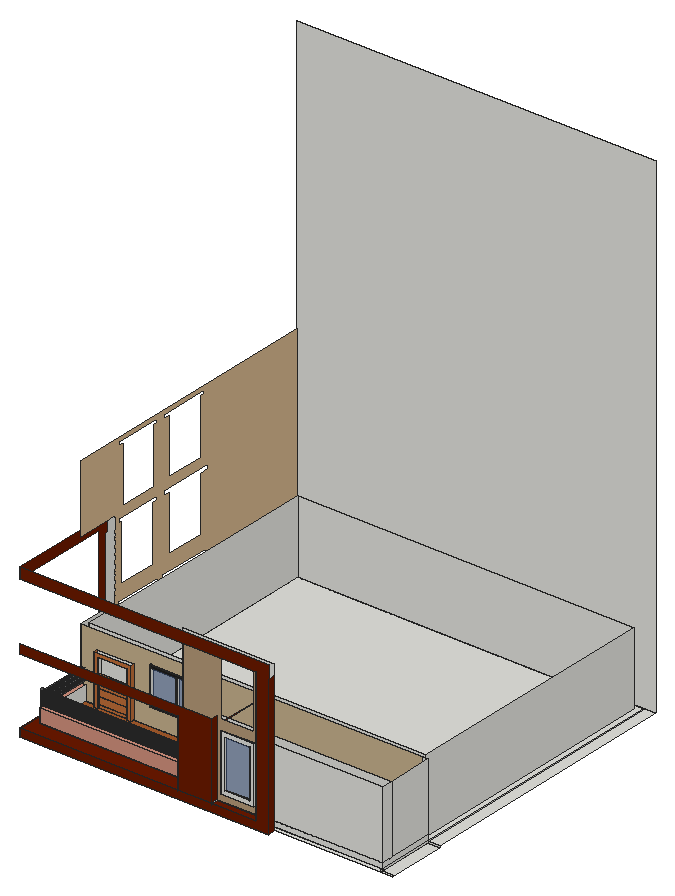
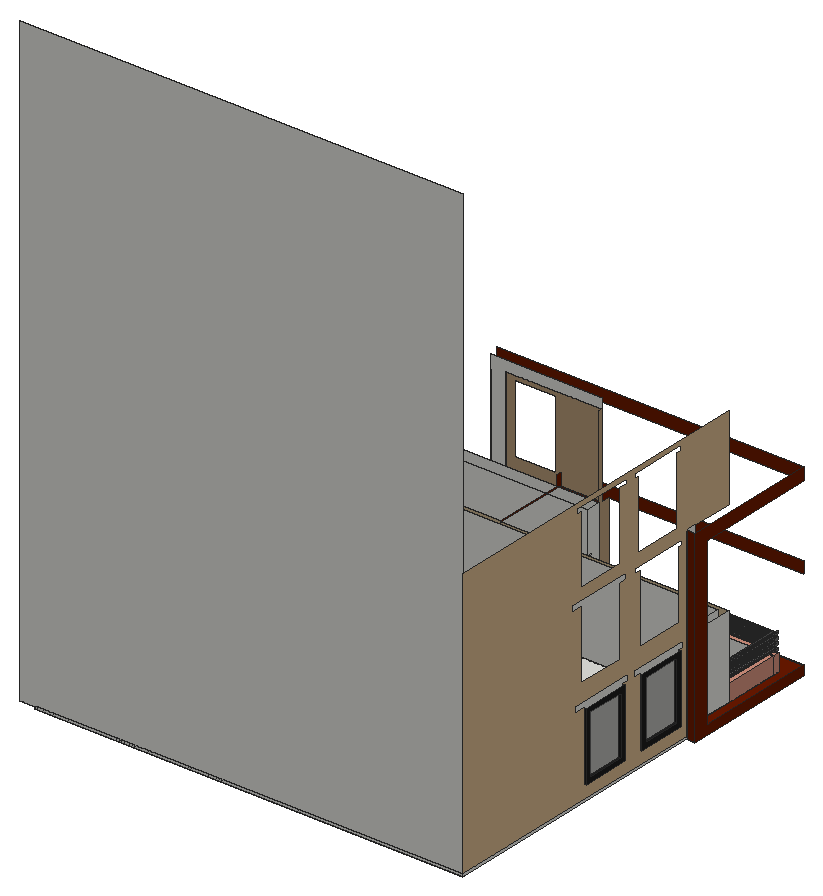
# SketchUp Ruby script. Lengths in inches.
U = 1.inch
M = Sketchup.active_model
def pt(a) = Geom::Point3d.new(a.map { |v| v * U })
def face(e, loops, mat)
  f = e.add_face(loops[0].map { |a| pt(a) })
  loops[1..].each { |l| e.add_face(l.map { |a| pt(a) }).erase! }
  f.material = f.back_material = mat if mat
  f
end
# faces: each face lists its corners as indices into pts; further lists are holes
def faces(e, pts, list, mat = nil) = list.each { |f| face(e, (f[0].is_a?(Array) ? f : [f]).map { |l| l.map { |i| pts[i] } }, mat) }
# xy, xz, yz: faces in a plane at the given z, y or x. An outline is a flat list of corners, or four numbers for a rectangle; further outlines are holes
def ring(l) = l.size == 4 ? [[l[0], l[1]], [l[2], l[1]], [l[2], l[3]], [l[0], l[3]]] : l.each_slice(2).to_a
def flat(e, list, mat, &to3) = list.each { |f| face(e, (f[0].is_a?(Array) ? f : [f]).map { |l| ring(l).map { |u, v| to3.(u, v) } }, mat) }
def xy(e, z, list, mat = nil) = flat(e, list, mat) { |x, y| [x, y, z] }
def xz(e, y, list, mat = nil) = flat(e, list, mat) { |x, z| [x, y, z] }
def yz(e, x, list, mat = nil) = flat(e, list, mat) { |y, z| [x, y, z] }
def lines(e, pts, list) = list.each { |a, b| e.add_line(pt(pts[a]), pt(pts[b])) }
# prism: a flat outline (further loops are holes) pulled along v
def prism(e, loops, v, mat = nil)
  f = face(e, loops, mat); d = Geom::Vector3d.new(v.map { |x| x * U })
  f.pushpull(f.normal.samedirection?(d) ? d.length : -d.length)
end
def box(e, o, s, mat = nil) = prism(e, [[o, [o[0] + s[0], o[1], o[2]], [o[0] + s[0], o[1] + s[1], o[2]], [o[0], o[1] + s[1], o[2]]]], [0, 0, s[2]], mat)
def at(x, y, z, deg = 0) = Geom::Transformation.translation(pt([x, y, z])) * Geom::Transformation.rotation(ORIGIN, Z_AXIS, deg.degrees)
def axes(o, x, y, z) = Geom::Transformation.new([*x, 0, *y, 0, *z, 0, *pt(o).to_a, 1])
def part(name) = M.definitions.add(name)
# library, detail: a bought-in or finely detailed component or shape, given as its bounding box
def library(name, o, s) = part(name).tap { |d| box(d.entities, o, s) }
def detail(e, o, s) = box(e.add_group.entities, o, s)
def put(e, d, t, mat = nil) = e.add_instance(d, t).tap { |i| i.material = mat if mat }
def group(e, t, mat = nil) = e.add_group.tap { |g| g.transformation = t; g.material = mat if mat }.entities
root = M.entities
M.materials.add("[0032_Moccasin]").color = [198, 177, 141]
M.materials.add("[0035_Tan]").color = [181, 154, 120]
M.materials.add("[0035_Tan]1").color = [210, 180, 140]
M.materials.add("[0134_DimGray]").color = [105, 105, 105]
M.materials.add("[Color B02]").color = [209, 145, 125]
M.materials.add("[Color B07]").color = [107, 26, 0]
M.materials.add("[Color M08]").color = [30, 30, 30]
M.materials.add("[Translucent Glass Blue]").color = [61, 91, 145]
M.materials["[Translucent Glass Blue]"].alpha = 0.5
M.materials.add("[Translucent Glass Gray]").color = [128, 128, 128]
M.materials["[Translucent Glass Gray]"].alpha = 0.5
M.materials.add("[Wood Square Tile 01]").color = [164, 91, 44]
M.materials.add("[Wood Veneer 01]").color = [191, 111, 58]
xy(root,123,[[[23.624,9.857,23.624,189.6875,34.874,189.6875,34.874,561.976,604.124,561.976,604.124,23.9375,299.436,23.9375,299.436,20.9375,430.624,20.9375,430.624,9.857],[542.499,503.926,551.499,532.164],[542.499,420.614,551.499,448.851],[542.499,52.1875,551.499,80.425]],[604.124,23.9375,622.998,26.9375],[604.124,26.9375,622.998,119.9375],[542.499,52.1875,551.499,80.425],[542.499,503.926,551.499,532.164]])
xy(root,126,[[34.874,26.9375,410.072,35.9375],[410.072,26.9375,410.072,35.9375,595.124,35.9375,595.124,119.9375,604.124,119.9375,604.124,26.9375],[34.874,35.9375,34.874,119.9375,61.398,119.9375,61.398,113.9375,67.398,113.9375,67.398,116.9375,115.398,116.9375,115.398,113.9375,121.398,113.9375,121.398,119.9375,595.124,119.9375,595.124,35.9375],[61.398,113.9375,67.398,119.9375],[115.398,113.9375,121.398,119.9375],
  [67.398,116.9375,115.398,119.9375],[34.874,119.9375,38.249,189.6875],[[38.249,119.9375,604.124,119.9375,604.124,561.976,34.874,561.976,34.874,189.6875,38.249,189.6875],[43.874,125.9375,595.124,552.976]],[604.124,119.9375,622.998,561.976],[43.874,125.9375,595.124,552.976]])
xy(root,134.528,[[282.124,16.419,337.624,20.9375],[282.124,20.9375,410.072,26.9375],[410.072,26.9375,604.124,26.9375,604.124,44.9375,595.124,44.9375,595.124,35.9375,410.072,35.9375],[410.072,35.9375,595.124,44.9375]])
xy(root,134.528,[[43.874,44.9375,604.124,44.9375,604.124,119.9375,121.398,119.9375,121.398,113.9375,115.398,113.9375,115.398,116.9375,67.398,116.9375,67.398,113.9375,61.398,113.9375,61.398,119.9375,43.874,119.9375]],"[Wood Square Tile 01]")
xy(root,136.146,[[282.124,9.857,337.624,20.9375],[282.124,26.9375,410.072,35.9375],[34.874,35.9375,38.249,44.9375],[38.249,35.9375,282.124,44.9375],[282.124,35.9375,410.072,44.9375]])
xy(root,136.146,[[23.624,9.857,282.124,9.857,282.124,35.9375,34.874,35.9375,34.874,170.669,23.624,170.669],[337.624,9.857,410.072,20.9375]],"[Color B07]")
xy(root,144.554,[[31.874,203.038,34.874,267.163],[31.874,295.913,34.874,360.038]],"[Color M08]")
xy(root,149.334,[[346.097,17.9375,399.784,20.9375]])
xy(root,150.554,[[31.874,209.038,34.874,261.163],[31.874,301.913,34.874,354.038]],"[Color M08]")
xy(root,155.334,[[352.097,17.9375,393.784,20.9375]])
xy(root,158.528,[[410.072,35.9375,595.124,44.9375]])
xy(root,158.528,[[34.874,35.9375,410.072,44.9375],[34.874,44.9375,43.874,119.9375]],"[Color B02]")
xy(root,165.189,[[149.96,116.9375,235.647,119.9375]])
xy(root,168.189,[[152.96,116.9375,192.804,119.9375],[195.804,116.9375,232.647,119.9375]])
xz(root,9.857,[[23.624,123,430.624,123,430.624,372,23.624,372,23.624,355.125,410.072,355.125,410.072,136.146,23.624,136.146],[282.124,136.146,337.624,136.146,337.624,260.108,23.624,260.108,23.624,244.827,282.124,244.827]],"[Color B07]")
xz(root,17.9375,[[[346.097,149.334,399.784,241.146],[352.097,155.334,393.784,235.146]]])
xz(root,20.9375,[[410.072,126,430.624,126,430.624,369,282.124,369,282.124,355.125,410.072,355.125],[282.124,134.528,337.624,136.146],[337.624,134.528,410.072,136.146],[[346.097,149.334,399.784,241.146],[352.097,155.334,393.784,235.146]]])
xz(root,20.9375,[[[337.624,136.146,410.072,136.146,410.072,355.125,282.124,355.125,282.124,244.827,337.624,244.827],[344.259,257.083,397.947,348.895],[346.097,149.334,399.784,241.146]]],"[0035_Tan]")
xz(root,20.9375,[[352.097,155.334,393.784,235.146]],"[Translucent Glass Blue]")
xz(root,26.9375,[[410.072,126,604.124,134.528],[282.124,134.528,410.072,136.146],[410.072,134.528,604.124,134.528,604.124,246,282.124,246,282.124,136.146,410.072,136.146]])
xz(root,35.9375,[[34.874,126,38.249,134.528],[38.249,126,410.072,134.528],[410.072,126,595.124,134.528],[34.874,134.528,38.249,136.146],[38.249,134.528,410.072,136.146],
  [410.072,134.528,595.124,158.528]])
xz(root,35.9375,[[34.874,136.146,410.072,158.528]],"[Color B02]")
xz(root,38.048,[[36.489,163.337,41.128,163.337,41.183,163.761,41.102,164.375,41.023,164.566,36.593,164.566,36.514,164.375,36.433,163.761]])
xz(root,38.048,[[38.808,161.386,39.423,161.466,39.996,161.704,40.488,162.081,40.865,162.573,41.102,163.146,41.128,163.337,36.489,163.337,36.514,163.146,36.752,162.573,37.129,162.081,37.621,161.704,38.194,161.466],[36.593,164.566,41.023,164.566,40.865,164.948,40.488,165.44,39.996,165.817,39.423,166.055,38.808,166.136,38.194,166.055,37.621,165.817,37.129,165.44,36.752,164.948]],"[0134_DimGray]")
xz(root,44.9375,[[43.874,134.528,410.072,136.146],[595.124,134.528,595.124,158.528,282.124,158.528,282.124,246,604.124,246,604.124,134.528],[410.072,134.528,595.124,158.528],[34.874,136.146,43.874,158.528],[43.874,136.146,282.124,158.528],
  [282.124,136.146,410.072,158.528]])
xz(root,113.9375,[[61.398,126,67.398,134.528],[115.398,126,121.398,134.528]])
xz(root,113.9375,[[61.398,134.528,67.398,134.528,67.398,210,115.398,210,115.398,134.528,121.398,134.528,121.398,216,61.398,216]],"[Wood Veneer 01]")
xz(root,116.9375,[[67.398,126,115.398,134.528],[67.398,139.025,115.398,139.942],[67.398,150.587,115.398,151.504],[67.398,162.15,115.398,163.067],[67.398,173.712,115.398,174.629]])
xz(root,116.9375,[[[149.96,165.189,235.647,225.876],[152.96,168.189,192.804,222.876],[195.804,168.189,232.647,222.876]]],"[Color M08]")
xz(root,116.9375,[[67.398,134.528,115.398,139.025],[67.398,139.942,115.398,150.587],[67.398,151.504,115.398,162.15],[67.398,163.067,115.398,173.712],[67.398,174.629,115.398,185.275]],"[Wood Veneer 01]")
xz(root,119.9375,[[604.124,123,622.998,126],[34.874,126,38.249,134.528],[38.249,126,61.398,134.528],[61.398,126,61.398,216,121.398,216,121.398,126,115.398,126,115.398,210,67.398,210,67.398,126],[67.398,126,115.398,210],
  [121.398,126,595.124,134.528],[595.124,126,604.124,134.528],[34.874,134.528,38.249,158.528],[38.249,134.528,43.874,158.528],[595.124,134.528,604.124,246],
  [[149.96,165.189,235.647,225.876],[152.96,168.189,192.804,222.876],[195.804,168.189,232.647,222.876]]])
xz(root,119.9375,[[[43.874,134.528,61.398,134.528,61.398,216,121.398,216,121.398,134.528,595.124,134.528,595.124,246,337.624,246,337.624,244.827,34.874,244.827,34.874,158.528,43.874,158.528],[149.96,165.189,235.647,225.876],[38.808,161.386,38.194,161.466,37.621,161.704,37.129,162.081,36.752,162.573,36.514,163.146,36.433,163.761,36.514,164.375,36.752,164.948,37.129,165.44,37.621,165.817,38.194,166.055,38.808,166.136,39.423,166.055,39.996,165.817,40.488,165.44,40.865,164.948,41.102,164.375,41.183,163.761,41.102,163.146,40.865,162.573,40.488,162.081,39.996,161.704,39.423,161.466]]],"[0032_Moccasin]")
xz(root,119.9375,[[152.96,168.189,192.804,222.876],[195.804,168.189,232.647,222.876]],"[Translucent Glass Blue]")
xz(root,125.9375,[[43.874,126,595.124,246]])
xz(root,170.669,[[23.624,134.528,34.874,136.146]])
xz(root,170.669,[[23.624,136.146,34.874,244.827]],"[Color B07]")
xz(root,189.6875,[[34.874,123,38.249,126]])
xz(root,189.6875,[[23.624,123,34.874,372]],"[Color B07]")
xz(root,203.038,[[31.874,144.554,34.874,234.992]],"[Color M08]")
xz(root,209.038,[[31.874,150.554,34.874,228.992]],"[Color M08]")
xz(root,261.163,[[31.874,150.554,34.874,228.992]],"[Color M08]")
xz(root,267.163,[[31.874,144.554,34.874,234.992]],"[Color M08]")
xz(root,295.913,[[31.874,144.554,34.874,234.992]],"[Color M08]")
xz(root,301.913,[[31.874,150.554,34.874,228.992]],"[Color M08]")
xz(root,354.038,[[31.874,150.554,34.874,228.992]],"[Color M08]")
xz(root,360.038,[[31.874,144.554,34.874,234.992]],"[Color M08]")
xz(root,420.614,[[542.499,123,551.499,126]])
xz(root,448.851,[[542.499,123,551.499,126]])
xz(root,503.926,[[542.499,123,551.499,123.5625],[542.499,123.5625,551.499,126]])
xz(root,532.164,[[542.499,123,551.499,123.5625],[542.499,123.5625,551.499,126]])
xz(root,552.976,[[43.874,126,595.124,246]])
xz(root,561.976,[[34.874,123,604.124,126],[34.874,126,622.998,936]])
yz(root,23.624,[[9.857,123,9.857,136.146,170.669,136.146,170.669,355.125,9.857,355.125,9.857,372,189.6875,372,189.6875,123]],"[Color B07]")
yz(root,31.874,[[[203.038,144.554,267.163,234.992],[209.038,150.554,261.163,228.992]],[[295.913,144.554,360.038,234.992],[301.913,150.554,354.038,228.992]]],"[Color M08]")
yz(root,34.874,[[189.6875,123,561.976,126],[35.9375,126,119.9375,136.146],[119.9375,126,189.6875,134.528],[119.9375,134.528,170.669,136.146],[170.669,134.528,189.6875,134.528,189.6875,372,175.544,372,175.544,355.125,170.669,355.125],
  [119.9375,136.146,170.669,244.827]])
yz(root,34.874,[[[189.6875,126,189.6875,372,119.9375,372,119.9375,483.875,561.976,483.875,561.976,126],[301.476,266.992,365.601,266.992,365.601,357.429,380.288,357.429,380.288,365.492,289.976,365.492,289.976,357.429,301.476,357.429],[295.913,144.554,360.038,144.554,360.038,234.992,375.601,234.992,375.601,242.929,286.991,242.929,286.991,234.992,295.913,234.992],[203.038,144.554,267.163,144.554,267.163,234.992,278.069,234.992,278.069,242.929,196.101,242.929,196.101,234.992,203.038,234.992],[301.476,380.367,365.601,380.367,365.601,470.804,372.101,470.804,372.101,477.304,289.663,477.304,289.663,470.804,301.476,470.804],[206.288,380.367,270.413,380.367,270.413,470.804,276.257,470.804,276.257,477.304,198.913,477.304,198.913,470.804,206.288,470.804],[203.038,266.992,267.163,266.992,267.163,357.429,275.257,357.429,275.257,363.742,198.038,363.742,198.038,357.429,203.038,357.429]]],"[0035_Tan]1")
yz(root,34.874,[[40.342,161.576,39.727,161.657,39.154,161.894,38.663,162.272,38.285,162.764,38.048,163.337,37.967,163.951,38.048,164.566,38.285,165.139,38.663,165.631,39.154,166.008,39.727,166.245,40.342,166.326,40.957,166.245,41.529,166.008,42.021,165.631,42.399,165.139,42.636,164.566,42.717,163.951,42.636,163.337,42.399,162.764,42.021,162.272,41.529,161.894,40.957,161.657],[40.342,168.076,39.727,168.157,39.154,168.394,38.663,168.772,38.285,169.264,38.048,169.837,37.967,170.451,38.048,171.066,38.285,171.639,38.663,172.131,39.154,172.508,39.727,172.745,40.342,172.826,40.957,172.745,41.529,172.508,42.021,172.131,42.399,171.639,42.636,171.066,42.717,170.451,42.636,169.837,42.399,169.264,42.021,168.772,41.529,168.394,40.957,168.157],[40.342,174.576,39.727,174.657,39.154,174.894,38.663,175.272,38.285,175.764,38.048,176.337,37.967,176.951,38.048,177.566,38.285,178.139,38.663,178.631,39.154,179.008,39.727,179.245,40.342,179.326,40.957,179.245,41.529,179.008,42.021,178.631,42.399,178.139,42.636,177.566,42.717,176.951,42.636,176.337,42.399,175.764,42.021,175.272,41.529,174.894,40.957,174.657],[40.342,181.076,39.727,181.157,39.154,181.394,38.663,181.772,38.285,182.264,38.048,182.837,37.967,183.451,38.048,184.066,38.285,184.639,38.663,185.131,39.154,185.508,39.727,185.745,40.342,185.826,40.957,185.745,41.529,185.508,42.021,185.131,42.399,184.639,42.636,184.066,42.717,183.451,42.636,182.837,42.399,182.264,42.021,181.772,41.529,181.394,40.957,181.157]],"[0134_DimGray]")
yz(root,34.874,[[35.9375,136.146,44.9375,158.528],[44.9375,136.146,119.9375,158.528]],"[Color B02]")
yz(root,34.874,[[209.038,150.554,261.163,228.992],[301.913,150.554,354.038,228.992]],"[Translucent Glass Gray]")
yz(root,43.874,[[125.9375,126,552.976,246],[44.9375,134.528,119.9375,158.528]])
yz(root,61.398,[[113.9375,126,119.9375,134.528]])
yz(root,61.398,[[113.9375,134.528,119.9375,216]],"[Wood Veneer 01]")
yz(root,67.398,[[113.9375,126,116.9375,134.528],[116.9375,126,119.9375,210]])
yz(root,67.398,[[113.9375,134.528,116.9375,210]],"[Wood Veneer 01]")
yz(root,115.398,[[113.9375,126,116.9375,134.528],[116.9375,126,119.9375,210]])
yz(root,115.398,[[113.9375,134.528,116.9375,210]],"[Wood Veneer 01]")
yz(root,121.398,[[113.9375,126,119.9375,134.528]])
yz(root,121.398,[[113.9375,134.528,119.9375,216]],"[Wood Veneer 01]")
yz(root,149.96,[[116.9375,165.189,119.9375,225.876]],"[Color M08]")
yz(root,152.96,[[116.9375,168.189,119.9375,222.876]])
yz(root,192.804,[[116.9375,168.189,119.9375,222.876]],"[Color M08]")
yz(root,195.804,[[116.9375,168.189,119.9375,222.876]])
yz(root,232.647,[[116.9375,168.189,119.9375,222.876]],"[Color M08]")
yz(root,235.647,[[116.9375,165.189,119.9375,225.876]])
yz(root,282.124,[[9.857,134.528,20.9375,136.146],[20.9375,134.528,26.9375,136.146],[[26.9375,136.146,44.9375,246],[40.342,161.576,40.957,161.657,41.529,161.894,42.021,162.272,42.399,162.764,42.636,163.337,42.717,163.951,42.636,164.566,42.399,165.139,42.021,165.631,41.529,166.008,40.957,166.245,40.342,166.326,39.727,166.245,39.154,166.008,38.663,165.631,38.285,165.139,38.048,164.566,37.967,163.951,38.048,163.337,38.285,162.764,38.663,162.272,39.154,161.894,39.727,161.657],[40.342,168.076,40.957,168.157,41.529,168.394,42.021,168.772,42.399,169.264,42.636,169.837,42.717,170.451,42.636,171.066,42.399,171.639,42.021,172.131,41.529,172.508,40.957,172.745,40.342,172.826,39.727,172.745,39.154,172.508,38.663,172.131,38.285,171.639,38.048,171.066,37.967,170.451,38.048,169.837,38.285,169.264,38.663,168.772,39.154,168.394,39.727,168.157],[40.342,174.576,40.957,174.657,41.529,174.894,42.021,175.272,42.399,175.764,42.636,176.337,42.717,176.951,42.636,177.566,42.399,178.139,42.021,178.631,41.529,179.008,40.957,179.245,40.342,179.326,39.727,179.245,39.154,179.008,38.663,178.631,38.285,178.139,38.048,177.566,37.967,176.951,38.048,176.337,38.285,175.764,38.663,175.272,39.154,174.894,39.727,174.657],[40.342,181.076,40.957,181.157,41.529,181.394,42.021,181.772,42.399,182.264,42.636,182.837,42.717,183.451,42.636,184.066,42.399,184.639,42.021,185.131,41.529,185.508,40.957,185.745,40.342,185.826,39.727,185.745,39.154,185.508,38.663,185.131,38.285,184.639,38.048,184.066,37.967,183.451,38.048,182.837,38.285,182.264,38.663,181.772,39.154,181.394,39.727,181.157],[40.342,187.576,40.957,187.657,41.529,187.894,42.021,188.272,42.399,188.764,42.636,189.337,42.717,189.951,42.636,190.566,42.399,191.139,42.021,191.631,41.529,192.008,40.957,192.245,40.342,192.326,39.727,192.245,39.154,192.008,38.663,191.631,38.285,191.139,38.048,190.566,37.967,189.951,38.048,189.337,38.285,188.764,38.663,188.272,39.154,187.894,39.727,187.657]]])
yz(root,282.124,[[9.857,136.146,9.857,244.827,20.9375,244.827,20.9375,355.125,26.9375,355.125,26.9375,136.146]],"[0035_Tan]")
yz(root,337.624,[[9.857,134.528,20.9375,136.146]])
yz(root,337.624,[[9.857,136.146,20.9375,136.146,20.9375,244.827,119.9375,244.827,119.9375,246,26.9375,246,26.9375,260.108,9.857,260.108]],"[Color B07]")
yz(root,346.097,[[17.9375,149.334,20.9375,241.146]])
yz(root,352.097,[[17.9375,155.334,20.9375,235.146]])
yz(root,393.784,[[17.9375,155.334,20.9375,235.146]])
yz(root,399.784,[[17.9375,149.334,20.9375,241.146]])
yz(root,410.072,[[20.9375,126,26.9375,134.528],[26.9375,126,35.9375,134.528],[26.9375,134.528,35.9375,136.146],[35.9375,134.528,44.9375,136.146],[35.9375,136.146,44.9375,158.528]])
yz(root,410.072,[[9.857,136.146,20.9375,355.125]],"[Color B07]")
yz(root,430.624,[[9.857,123,20.9375,350.472]],"[Color B07]")
yz(root,542.499,[[420.614,123,448.851,123.5625],[503.926,123,532.164,123.5625],[420.614,123.5625,448.851,126],[503.926,123.5625,532.164,126]])
yz(root,551.499,[[420.614,123,448.851,126],[503.926,123,532.164,126]])
yz(root,595.124,[[125.9375,126,552.976,246],[35.9375,134.528,44.9375,158.528]])
yz(root,604.124,[[23.9375,123,26.9375,126],[26.9375,123,119.9375,126],[119.9375,123,561.976,126],[26.9375,126,119.9375,134.528],[26.9375,134.528,44.9375,246],
  [44.9375,134.528,119.9375,246]])
p = [[38.194,119.9375,161.466],[38.808,119.9375,161.386],[38.808,38.048,161.386],[38.194,38.048,161.466],[39.423,119.9375,161.466],[39.423,38.048,161.466],
  [37.621,119.9375,161.704],[37.621,38.048,161.704],[39.996,119.9375,161.704],[39.996,38.048,161.704],[282.124,40.342,161.576],[282.124,39.727,161.657],
  [34.874,39.727,161.657],[34.874,40.342,161.576],[282.124,40.957,161.657],[34.874,40.957,161.657],[37.129,119.9375,162.081],[37.129,38.048,162.081],
  [40.488,119.9375,162.081],[40.488,38.048,162.081],[282.124,39.154,161.894],[34.874,39.154,161.894],[282.124,41.529,161.894],[34.874,41.529,161.894],
  [282.124,38.663,162.272],[34.874,38.663,162.272],[282.124,42.021,162.272],[34.874,42.021,162.272],[36.752,119.9375,162.573],[36.752,38.048,162.573],
  [40.865,119.9375,162.573],[40.865,38.048,162.573],[282.124,38.285,162.764],[34.874,38.285,162.764],[282.124,42.399,162.764],[34.874,42.399,162.764],
  [36.514,119.9375,163.146],[36.514,38.048,163.146],[41.102,119.9375,163.146],[41.102,38.048,163.146],[282.124,38.048,163.337],[41.128,38.048,163.337],
  [36.489,38.048,163.337],[34.874,38.048,163.337],[282.124,42.636,163.337],[34.874,42.636,163.337],[36.433,119.9375,163.761],[36.433,38.048,163.761],
  [41.183,119.9375,163.761],[41.183,38.048,163.761],[282.124,37.967,163.951],[34.874,37.967,163.951],[282.124,42.717,163.951],[34.874,42.717,163.951],
  [36.514,119.9375,164.375],[36.514,38.048,164.375],[41.102,119.9375,164.375],[41.102,38.048,164.375],[282.124,38.048,164.566],[41.023,38.048,164.566],
  [36.593,38.048,164.566],[34.874,38.048,164.566],[282.124,42.636,164.566],[34.874,42.636,164.566],[36.752,119.9375,164.948],[36.752,38.048,164.948],
  [40.865,119.9375,164.948],[40.865,38.048,164.948],[282.124,38.285,165.139],[34.874,38.285,165.139],[282.124,42.399,165.139],[34.874,42.399,165.139],
  [37.129,119.9375,165.44],[37.129,38.048,165.44],[40.488,119.9375,165.44],[40.488,38.048,165.44],[282.124,38.663,165.631],[34.874,38.663,165.631],
  [282.124,42.021,165.631],[34.874,42.021,165.631],[37.621,119.9375,165.817],[37.621,38.048,165.817],[39.996,119.9375,165.817],[39.996,38.048,165.817],
  [282.124,39.154,166.008],[34.874,39.154,166.008],[282.124,41.529,166.008],[34.874,41.529,166.008],[38.194,119.9375,166.055],[38.194,38.048,166.055],
  [39.423,119.9375,166.055],[39.423,38.048,166.055],[282.124,39.727,166.245],[34.874,39.727,166.245],[282.124,40.957,166.245],[34.874,40.957,166.245],
  [38.808,119.9375,166.136],[38.808,38.048,166.136],[282.124,40.342,166.326],[34.874,40.342,166.326],[38.194,119.9375,168.216],[38.808,119.9375,168.136],
  [38.808,38.048,168.136],[38.194,38.048,168.216],[39.423,119.9375,168.216],[39.423,38.048,168.216],[282.124,40.342,168.076],[282.124,39.727,168.157],
  [34.874,39.727,168.157],[34.874,40.342,168.076],[282.124,40.957,168.157],[34.874,40.957,168.157],[37.621,119.9375,168.454],[37.621,38.048,168.454],
  [39.996,119.9375,168.454],[39.996,38.048,168.454],[282.124,39.154,168.394],[34.874,39.154,168.394],[282.124,41.529,168.394],[34.874,41.529,168.394],
  [282.124,38.663,168.772],[34.874,38.663,168.772],[282.124,42.021,168.772],[34.874,42.021,168.772],[37.129,119.9375,168.831],[37.129,38.048,168.831],
  [40.488,119.9375,168.831],[40.488,38.048,168.831],[36.752,119.9375,169.323],[36.752,38.048,169.323],[40.865,119.9375,169.323],[40.865,38.048,169.323],
  [282.124,38.285,169.264],[34.874,38.285,169.264],[282.124,42.399,169.264],[34.874,42.399,169.264],[282.124,38.048,169.837],[41.078,38.048,169.837],
  [36.539,38.048,169.837],[34.874,38.048,169.837],[36.514,119.9375,169.896],[36.514,38.048,169.896],[41.102,119.9375,169.896],[41.102,38.048,169.896],
  [282.124,42.636,169.837],[34.874,42.636,169.837],[282.124,37.967,170.451],[34.874,37.967,170.451],[282.124,42.717,170.451],[34.874,42.717,170.451],
  [36.433,119.9375,170.511],[36.489,38.048,170.087],[36.433,38.048,170.511],[41.183,119.9375,170.511],[41.183,38.048,170.511],[41.128,38.048,170.087],
  [282.124,38.048,171.066],[41.11,38.048,171.066],[36.507,38.048,171.066],[34.874,38.048,171.066],[36.514,119.9375,171.125],[36.514,38.048,171.125],
  [41.102,119.9375,171.125],[41.102,38.048,171.125],[282.124,42.636,171.066],[34.874,42.636,171.066],[282.124,38.285,171.639],[34.874,38.285,171.639],
  [36.752,119.9375,171.698],[36.593,38.048,171.316],[36.752,38.048,171.698],[40.865,119.9375,171.698],[40.865,38.048,171.698],[41.023,38.048,171.316],
  [282.124,42.399,171.639],[34.874,42.399,171.639],[282.124,38.663,172.131],[34.874,38.663,172.131],[282.124,42.021,172.131],[34.874,42.021,172.131],
  [37.129,119.9375,172.19],[37.129,38.048,172.19],[40.488,119.9375,172.19],[40.488,38.048,172.19],[282.124,39.154,172.508],[34.874,39.154,172.508],
  [282.124,41.529,172.508],[34.874,41.529,172.508],[37.621,119.9375,172.567],[37.621,38.048,172.567],[39.996,119.9375,172.567],[39.996,38.048,172.567],
  [282.124,39.727,172.745],[34.874,39.727,172.745],[282.124,40.957,172.745],[34.874,40.957,172.745],[38.194,119.9375,172.805],[38.194,38.048,172.805],
  [39.423,119.9375,172.805],[39.423,38.048,172.805],[282.124,40.342,172.826],[34.874,40.342,172.826],[38.808,119.9375,172.886],[38.808,38.048,172.886],
  [282.124,40.342,174.576],[282.124,39.727,174.657],[34.874,39.727,174.657],[34.874,40.342,174.576],[282.124,40.957,174.657],[34.874,40.957,174.657],
  [282.124,39.154,174.894],[34.874,39.154,174.894],[282.124,41.529,174.894],[34.874,41.529,174.894],[282.124,38.663,175.272],[34.874,38.663,175.272],
  [282.124,42.021,175.272],[34.874,42.021,175.272],[282.124,38.285,175.764],[34.874,38.285,175.764],[282.124,42.399,175.764],[34.874,42.399,175.764],
  [38.194,119.9375,175.716],[38.808,119.9375,175.636],[38.808,38.048,175.636],[38.194,38.048,175.716],[39.423,119.9375,175.716],[39.423,38.048,175.716],
  [37.621,119.9375,175.954],[37.621,38.048,175.954],[39.996,119.9375,175.954],[39.996,38.048,175.954],[282.124,38.048,176.337],[40.492,38.048,176.337],
  [37.125,38.048,176.337],[34.874,38.048,176.337],[282.124,42.636,176.337],[34.874,42.636,176.337],[37.129,119.9375,176.331],[37.129,38.048,176.331],
  [40.488,119.9375,176.331],[40.488,38.048,176.331],[282.124,37.967,176.951],[34.874,37.967,176.951],[36.752,119.9375,176.823],[36.752,38.048,176.823],
  [40.865,119.9375,176.823],[40.865,38.048,176.823],[282.124,42.717,176.951],[34.874,42.717,176.951],[36.514,119.9375,177.396],[36.539,38.048,177.337],
  [36.514,38.048,177.396],[41.102,119.9375,177.396],[41.102,38.048,177.396],[41.078,38.048,177.337],[282.124,38.048,177.566],[41.125,38.048,177.566],
  [36.492,38.048,177.566],[34.874,38.048,177.566],[282.124,42.636,177.566],[34.874,42.636,177.566],[36.433,119.9375,178.011],[36.489,38.048,177.587],
  [36.433,38.048,178.011],[41.183,119.9375,178.011],[41.183,38.048,178.011],[41.128,38.048,177.587],[282.124,38.285,178.139],[34.874,38.285,178.139],
  [282.124,42.399,178.139],[34.874,42.399,178.139],[36.514,119.9375,178.625],[36.507,38.048,178.566],[36.514,38.048,178.625],[41.102,119.9375,178.625],
  [41.102,38.048,178.625],[41.11,38.048,178.566],[282.124,38.663,178.631],[34.874,38.663,178.631],[282.124,42.021,178.631],[34.874,42.021,178.631],
  [36.752,119.9375,179.198],[36.593,38.048,178.816],[36.752,38.048,179.198],[40.865,119.9375,179.198],[40.865,38.048,179.198],[41.023,38.048,178.816],
  [282.124,39.154,179.008],[34.874,39.154,179.008],[282.124,41.529,179.008],[34.874,41.529,179.008],[282.124,39.727,179.245],[34.874,39.727,179.245],
  [282.124,40.957,179.245],[34.874,40.957,179.245],[37.129,119.9375,179.69],[37.129,38.048,179.69],[40.488,119.9375,179.69],[40.488,38.048,179.69],
  [282.124,40.342,179.326],[34.874,40.342,179.326],[37.621,119.9375,180.067],[37.621,38.048,180.067],[39.996,119.9375,180.067],[39.996,38.048,180.067],
  [38.194,119.9375,180.305],[38.194,38.048,180.305],[39.423,119.9375,180.305],[39.423,38.048,180.305],[38.808,119.9375,180.386],[38.808,38.048,180.386],
  [38.194,119.9375,181.091],[38.808,119.9375,181.011],[38.808,38.048,181.011],[38.194,38.048,181.091],[39.423,119.9375,181.091],[39.423,38.048,181.091],
  [37.621,119.9375,181.329],[37.621,38.048,181.329],[39.996,119.9375,181.329],[39.996,38.048,181.329],[282.124,40.342,181.076],[282.124,39.727,181.157],
  [34.874,39.727,181.157],[34.874,40.342,181.076],[282.124,40.957,181.157],[34.874,40.957,181.157],[282.124,39.154,181.394],[34.874,39.154,181.394],
  [282.124,41.529,181.394],[34.874,41.529,181.394],[37.129,119.9375,181.706],[37.129,38.048,181.706],[40.488,119.9375,181.706],[40.488,38.048,181.706],
  [282.124,38.663,181.772],[34.874,38.663,181.772],[282.124,42.021,181.772],[34.874,42.021,181.772],[36.752,119.9375,182.198],[37.125,38.048,181.712],
  [36.752,38.048,182.198],[40.865,119.9375,182.198],[40.865,38.048,182.198],[40.492,38.048,181.712],[282.124,38.285,182.264],[34.874,38.285,182.264],
  [282.124,42.399,182.264],[34.874,42.399,182.264],[36.514,119.9375,182.771],[36.539,38.048,182.712],[36.514,38.048,182.771],[41.102,119.9375,182.771],
  [41.102,38.048,182.771],[41.078,38.048,182.712],[282.124,38.048,182.837],[41.111,38.048,182.837],[36.506,38.048,182.837],[34.874,38.048,182.837],
  [282.124,42.636,182.837],[34.874,42.636,182.837],[542.499,80.425,123],[540.561,80.425,123],[71.499,80.101,123.75],[71.499,52.1875,123.75],
  [604.124,26.9375,126],[607.124,26.9375,126],[282.124,26.9375,134.528],[282.124,26.9375,126],[551.499,80.425,123],[551.499,80.425,126],
  [542.499,61.1875,123],[542.499,61.1875,126],[542.499,52.1875,123],[542.499,52.1875,126],[38.249,35.9375,126],[38.249,35.9375,123],
  [604.124,23.9375,123],[604.124,20.9375,123]]
faces(root,p,[[0,1,2,3],[1,4,5,2],[6,0,3,7],[4,8,9,5],[10,11,12,13],[14,10,13,15],[16,6,7,17],[8,18,19,9],
  [11,20,21,12],[22,14,15,23],[20,24,25,21],[26,22,23,27],[28,16,17,29],[18,30,31,19],[24,32,33,25],[34,26,27,35],
  [36,28,29,37],[30,38,39,31],[32,40,41,42,43,33],[44,34,35,45],[46,36,37,42,47],[38,48,49,41,39],[40,50,51,43,42,41],[52,44,45,53],
  [54,46,47,55],[48,56,57,49],[50,58,59,60,61,51],[62,52,53,63],[64,54,55,60,65],[56,66,67,59,57],[58,68,69,61,60,59],[70,62,63,71],
  [72,64,65,73],[66,74,75,67],[68,76,77,69],[78,70,71,79],[80,72,73,81],[74,82,83,75],[76,84,85,77],[86,78,79,87],
  [88,80,81,89],[82,90,91,83],[84,92,93,85],[94,86,87,95],[96,88,89,97],[90,96,97,91],[92,98,99,93],[98,94,95,99],
  [100,101,102,103],[101,104,105,102],[106,107,108,109],[110,106,109,111],[112,100,103,113],[104,114,115,105],[107,116,117,108],[118,110,111,119],
  [116,120,121,117],[122,118,119,123],[124,112,113,125],[114,126,127,115],[128,124,125,129],[126,130,131,127],[120,132,133,121],[134,122,123,135],
  [132,136,137,138,139,133],[140,128,129,138,141],[130,142,143,137,131],[144,134,135,145],[136,146,147,139,138,137],[148,144,145,149],[150,140,141,151,152],[142,153,154,155,143],
  [146,156,157,158,159,147],[160,150,152,158,161],[153,162,163,157,154],[164,148,149,165],[156,166,167,159,158,157],[168,160,161,169,170],[162,171,172,173,163],[174,164,165,175],
  [166,176,177,167],[178,174,175,179],[180,168,170,181],[171,182,183,172],[176,184,185,177],[186,178,179,187],[188,180,181,189],[182,190,191,183],
  [184,192,193,185],[194,186,187,195],[196,188,189,197],[190,198,199,191],[192,200,201,193],[200,194,195,201],[202,196,197,203],[198,202,203,199],
  [204,205,206,207],[208,204,207,209],[205,210,211,206],[212,208,209,213],[210,214,215,211],[216,212,213,217],[214,218,219,215],[220,216,217,221],
  [222,223,224,225],[223,226,227,224],[228,222,225,229],[226,230,231,227],[218,232,233,234,235,219],[236,220,221,237],[238,228,229,239],[230,240,241,231],
  [232,242,243,235,234,233],[244,238,239,234,245],[240,246,247,233,241],[248,236,237,249],[250,244,245,251,252],[246,253,254,255,247],[242,256,257,258,259,243],[260,248,249,261],
  [262,250,252,258,263,264],[253,265,266,267,257,254],[256,268,269,259,258,257],[270,260,261,271],[272,262,264,273,274],[265,275,276,277,266],[268,278,279,269],[280,270,271,281],
  [282,272,274,283,284],[275,285,286,287,276],[278,288,289,279],[290,280,281,291],[288,292,293,289],[294,290,291,295],[296,282,284,297],[285,298,299,286],
  [292,300,301,293],[300,294,295,301],[302,296,297,303],[298,304,305,299],[306,302,303,307],[304,308,309,305],[310,306,307,311],[308,310,311,309],
  [312,313,314,315],[313,316,317,314],[318,312,315,319],[316,320,321,317],[322,323,324,325],[326,322,325,327],[323,328,329,324],[330,326,327,331],
  [332,318,319,333],[320,334,335,321],[328,336,337,329],[338,330,331,339],[340,332,333,341,342],[334,343,344,345,335],[336,346,347,337],[348,338,339,349],
  [350,340,342,351,352],[343,353,354,355,344],[346,356,357,358,359,347],[360,348,349,361]],"[0134_DimGray]")
lines(root,p,[[362,363],[364,365],[366,367],[368,369],[370,371],[372,373],[374,375],[376,377],[378,379]])
